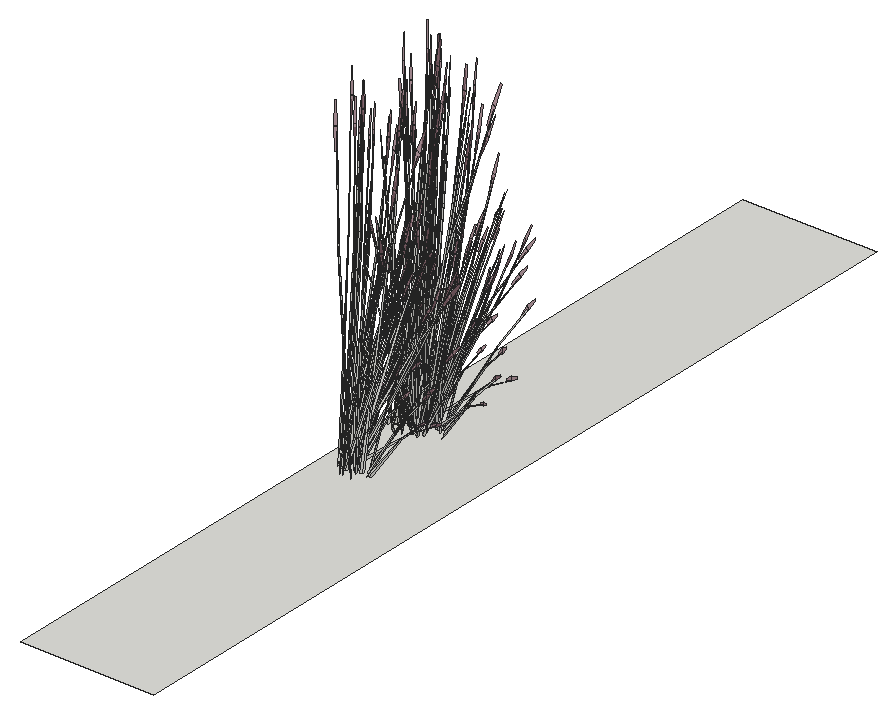
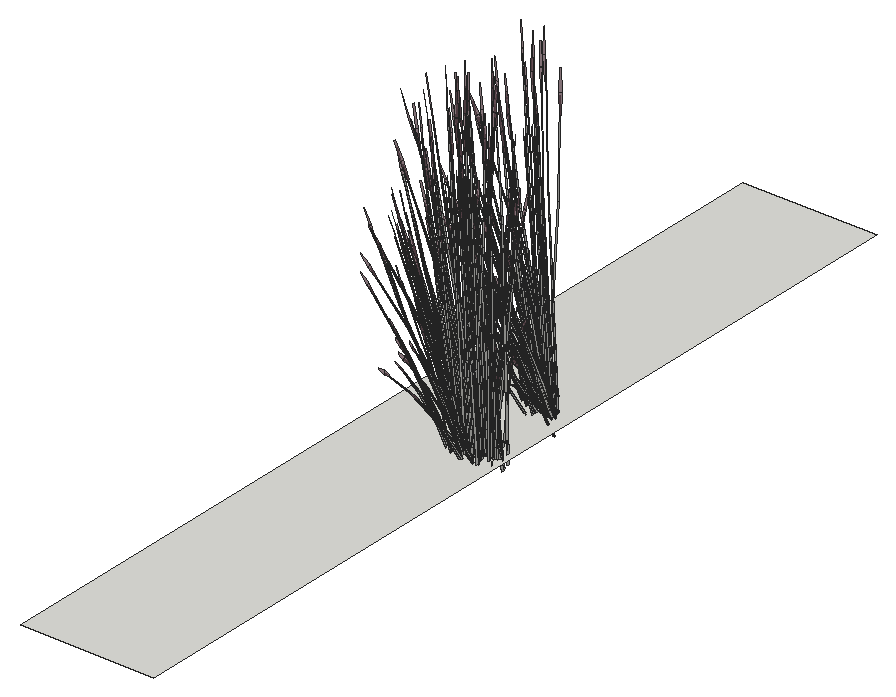
# SketchUp Ruby script. Lengths in inches.
U = 1.inch
M = Sketchup.active_model
def pt(a) = Geom::Point3d.new(a.map { |v| v * U })
def face(e, loops, mat)
  f = e.add_face(loops[0].map { |a| pt(a) })
  loops[1..].each { |l| e.add_face(l.map { |a| pt(a) }).erase! }
  f.material = f.back_material = mat if mat
  f
end
# faces: each face lists its corners as indices into pts; further lists are holes
def faces(e, pts, list, mat = nil) = list.each { |f| face(e, (f[0].is_a?(Array) ? f : [f]).map { |l| l.map { |i| pts[i] } }, mat) }
# xy, xz, yz: faces in a plane at the given z, y or x. An outline is a flat list of corners, or four numbers for a rectangle; further outlines are holes
def ring(l) = l.size == 4 ? [[l[0], l[1]], [l[2], l[1]], [l[2], l[3]], [l[0], l[3]]] : l.each_slice(2).to_a
def flat(e, list, mat, &to3) = list.each { |f| face(e, (f[0].is_a?(Array) ? f : [f]).map { |l| ring(l).map { |u, v| to3.(u, v) } }, mat) }
def xy(e, z, list, mat = nil) = flat(e, list, mat) { |x, y| [x, y, z] }
def xz(e, y, list, mat = nil) = flat(e, list, mat) { |x, z| [x, y, z] }
def yz(e, x, list, mat = nil) = flat(e, list, mat) { |y, z| [x, y, z] }
def lines(e, pts, list) = list.each { |a, b| e.add_line(pt(pts[a]), pt(pts[b])) }
# prism: a flat outline (further loops are holes) pulled along v
def prism(e, loops, v, mat = nil)
  f = face(e, loops, mat); d = Geom::Vector3d.new(v.map { |x| x * U })
  f.pushpull(f.normal.samedirection?(d) ? d.length : -d.length)
end
def box(e, o, s, mat = nil) = prism(e, [[o, [o[0] + s[0], o[1], o[2]], [o[0] + s[0], o[1] + s[1], o[2]], [o[0], o[1] + s[1], o[2]]]], [0, 0, s[2]], mat)
def at(x, y, z, deg = 0) = Geom::Transformation.translation(pt([x, y, z])) * Geom::Transformation.rotation(ORIGIN, Z_AXIS, deg.degrees)
def axes(o, x, y, z) = Geom::Transformation.new([*x, 0, *y, 0, *z, 0, *pt(o).to_a, 1])
def part(name) = M.definitions.add(name)
# library, detail: a bought-in or finely detailed component or shape, given as its bounding box
def library(name, o, s) = part(name).tap { |d| box(d.entities, o, s) }
def detail(e, o, s) = box(e.add_group.entities, o, s)
def put(e, d, t, mat = nil) = e.add_instance(d, t).tap { |i| i.material = mat if mat }
def group(e, t, mat = nil) = e.add_group.tap { |g| g.transformation = t; g.material = mat if mat }.entities
root = M.entities
M.materials.add("LightPink_Translucent").color = [144, 107, 117]
M.materials["LightPink_Translucent"].alpha = 0.75
c1 = part("blade")
p = [[2.15,0.21,22],[0,0.17,0],[0.09,0.45,0],[2.18,0.31,22],[2.29,0.31,22],[0.38,0.45,0],
  [2.48,0.24,33],[2.49,0.24,33],[2.48,0.22,33]]
faces(c1.entities,p,[[0,1,2,3],[4,5,2,3],[6,3,4,7],[8,0,3,6]])
c2 = part("seeds")
p = [[0.3,-0.1,1.38],[-0.01,-0.03,1.59],[-0.01,-0.03,0.03],[0.14,-0.07,-0.07],[0.29,-0.03,3],[0.15,0.01,3.11]]
faces(c2.entities,p,[[0,1,2,3],[1,0,4,5]],"LightPink_Translucent")
c3 = part("blade with seeds")
put(c3.entities,c1,at(0,0,0))
put(c3.entities,c2,axes([2.4,0.25,30.99],[1.5799,-0.05474,1.17369],[-0.12525,1.92788,0.29478],[-0.07173,-0.02425,1.56792]))
xy(root,6,[[342,51,366,213]])
put(root,c3,axes([345.73,119.64,4.48],[0.93921,-0.22138,-0.19198],[0.33003,0.6377,0.00008],[0.10367,-0.02447,1.73897]))
put(root,c3,axes([345.84,118.43,4.51],[0.62448,0.42144,0],[-0.62448,0.42144,0],[0,0,1.69266]))
put(root,c3,axes([347.53,118.25,4.77],[-0.70288,-0.47526,0.17642],[0.70832,-0.46097,0.35086],[-0.07763,0.09706,1.60407]))
put(root,c3,axes([346.23,117.53,4.35],[0.9306,0.10697,-0.62353],[-0.19638,0.65984,-0.16365],[0.27771,0.07995,1.37633]))
put(root,c3,axes([350.34,118.68,5.06],[-0.55274,0.10771,1.1486],[0.26018,-0.44517,0.84392],[0.29323,0.03046,0.25299]))
put(root,c3,axes([345.83,117.9375,5.01],[0.43405,-0.58792,0.44739],[0.90188,0.28295,-0.21531],[0,0.13553,1.43643]))
put(root,c3,axes([350.09,120.57,7],[-0.08089,-0.05712,1.77383],[0.17695,-0.61228,-0.16761],[0.31864,-0.03912,0.31391]))
put(root,c3,axes([345.67,118.28,4.59],[0,0.75458,-0.05637],[-1.11865,0,0],[0,0.02371,1.79368]))
put(root,c3,axes([345.75,117.74,4.5],[0.53742,0.54764,-0.44739],[-0.81403,0.38564,0.21531],[0.17391,0.06776,1.43643]))
put(root,c3,axes([349.38,120.06,6.22],[-0.17122,-0.54847,-0.03492],[0.80929,-0.12609,-0.15832],[0.169,0.03477,0.52218]))
put(root,c3,axes([347.28,120.04,7.33],[0.0479,-0.66354,-0.1216],[0.90696,0.01814,-0.67495],[0.3493,0.04609,1.02557]))
put(root,c3,axes([348.11,118.27,4.77],[0,-0.65246,0.49651],[1.00089,0,0],[0,0.1486,1.57504]))
put(root,c3,axes([346.21,118.07,4.91],[0.83351,-0.19028,0.1448],[0.29189,0.54335,-0.41347],[0,0.11958,1.26744]))
put(root,c3,axes([347.14,119.78,7.34],[-0.50902,-0.40851,0.35414],[0.58122,-0.38671,-0.4572],[0.29531,0.05884,0.87481]))
put(root,c3,axes([349.31,119.4,4.88],[-0.21545,-0.16047,1.43002],[0.28033,-0.53085,-0.30754],[0.43591,0.07191,0.61141]))
put(root,c3,axes([345.45,119.98,4.5],[0.90188,0.29293,0],[-0.43405,0.60866,0],[0,0,1.74954]))
put(root,c3,axes([348.07,119.64,7.01],[0.19191,-0.01103,1.74944],[0.52639,-0.5069,-0.27667],[0.34136,0.06691,0.14031]))
put(root,c3,axes([347.33,119.72,7.27],[0.89428,0.01571,-0.71045],[-0.06006,0.66153,0.08574],[0.37886,0.06981,1.00501]))
put(root,c3,axes([345.13,119.74,4.58],[0.38895,0.74956,-0.06012],[-1.11135,0.26265,0],[0.01358,0.02618,1.72173]))
put(root,c3,axes([348.79,118.38,4.67],[1.11865,0,0],[0,0.72922,-0.51607],[0,0.16609,1.63711]))
put(root,c3,axes([348.34,118.75,4.49],[-1.1181,-0.00522,-0.04976],[0,-0.72922,0.49943],[-0.03514,0.166,1.58352]))
put(root,c3,axes([345.92,118.12,4.96],[1.00749,0.31132,-0.29095],[-0.48511,0.65709,-0.50002],[0.03166,0.16133,1.59708]))
put(root,c3,axes([347.87,119.99,6.82],[0.50902,0.40851,-0.35414],[-0.58122,0.38671,0.4572],[0.29531,0.05884,0.87481]))
put(root,c3,axes([348.11,118.86,4.32],[-0.62448,0.40708,-0.30978],[-0.62448,-0.40708,0.30978],[0,0.13112,1.38974]))
put(root,c3,axes([347.61,120.15,7.02],[-0.04505,0.49615,0.0643],[-0.68022,-0.0136,0.50621],[0.26056,0.05192,0.77189]))
put(root,c3,axes([345.81,118.61,4.5],[-0.43405,0.58792,-0.44739],[-0.90188,-0.28295,0.21531],[0,0.13553,1.43643]))
put(root,c3,axes([347.67,119.99,7.03],[-0.65964,0.42992,0.48003],[-0.5689,-0.45657,0.3958],[0.30948,0.0793,0.9933]))
put(root,c3,axes([345.57,120.49,7.34],[-0.13817,-0.52554,0.35414],[0.78985,-0.13877,-0.4572],[0.21215,0.1506,0.87481]))
put(root,c3,axes([348.54,118.87,4.3125],[0,0.65246,-0.49651],[-1.00089,0,0],[0,0.1486,1.57504]))
put(root,c3,axes([346.04,118.95,6.17],[-0.3323,-0.11241,1.71376],[0.68769,-0.4716,0.13857],[0.42861,0.21275,0.73262]))
put(root,c3,axes([346.1,117.47,6.77],[-0.77304,-0.33901,1.38283],[0.81626,-0.52782,0.59665],[0.24941,0.31809,1.33663]))
put(root,c3,axes([347.27,120.23,5.06],[-0.5037,-0.18761,1.1486],[0.6504,-0.19062,0.84392],[0.17543,0.16147,0.25299]))
put(root,c3,axes([345.5,120.76,7.33],[0.53309,-0.55848,-0.1216],[0.77201,0.32175,-0.67495],[0.26836,0.15779,1.02557]))
put(root,c3,axes([344.8,121.23,7],[0.00265,-0.07899,1.77383],[0.76665,-0.34851,-0.16761],[0.2663,0.12439,0.31391]))
put(root,c3,axes([347.41,120.92,3.79],[0.06518,-0.0942,1.76342],[0.82057,-0.27742,-0.26939],[0.24877,0.14358,0.30037]))
put(root,c3,axes([346.33,118.78,4.39],[0.32803,0.59738,-0.69212],[-0.94492,0.21515,-0.18165],[0.03626,0.20229,1.52773]))
put(root,c3,axes([346.13,120.48,6.97],[0.88277,-0.1551,-0.51099],[0.15442,0.58737,-0.3958],[0.23711,0.16832,0.97773]))
put(root,c3,axes([343.68,120.57,7.34],[0.2697,-0.50175,0.35414],[0.78684,0.14635,-0.4572],[0.07215,0.20201,0.87481]))
put(root,c3,axes([347.35,121.08,4.96],[-0.57368,-0.02046,1.0506],[0.37886,-0.43461,0.58006],[0.22663,0.15441,0.8241]))
put(root,c3,axes([345.7,120.97,7.02],[-0.4066,0.41448,0.0643],[-0.57901,-0.24131,0.50621],[0.18719,0.13288,0.77189]))
put(root,c3,axes([344.74,122.36,7.9375],[0.61821,-0.37431,-0.06488],[0.56645,0.40995,-0.29416],[0.03988,0.11616,0.97024]))
put(root,c3,axes([345.87,120.85,7.03],[-0.88979,0.14973,0.48003],[-0.15442,-0.58737,0.3958],[0.20926,0.17311,0.9933]))
put(root,c3,axes([345.48,120.03,4.88],[0.01579,-0.21629,1.43002],[0.75442,-0.24159,-0.30754],[0.23289,0.25887,0.61141]))
put(root,c3,axes([343.42,120.78,7.33],[0.87543,-0.30377,-0.1216],[0.4302,0.53915,-0.67495],[0.1155,0.2272,1.02557]))
put(root,c3,axes([343.58,120.9,3.79],[0.14478,-0.0355,1.76342],[0.8709,0.19542,-0.26939],[0.02547,0.22025,0.30037]))
put(root,c3,axes([344.17,120.76,6.97],[0.87941,0.16356,-0.51099],[-0.30143,0.56078,-0.3958],[0.08064,0.22578,0.97773]))
put(root,c3,axes([344.67,119.6,6.17],[-0.2045,-0.20949,1.71376],[0.94495,-0.17636,0.13857],[0.21357,0.32887,0.73262]))
put(root,c3,axes([343.77,121.1,6.82],[-0.2697,0.50175,-0.35414],[-0.78684,-0.14635,0.4572],[0.07215,0.20201,0.87481]))
put(root,c3,axes([343.85,120.65,7.27],[0.42698,0.53052,-0.71045],[-0.87893,0.29566,0.08574],[0.09984,0.25633,1.00501]))
put(root,c3,axes([343.21,121.99,7.01],[0.1134,0.10507,1.74944],[0.91515,0.04128,-0.27667],[0.09203,0.23172,0.14031]))
put(root,c3,axes([346.1,132.13,4.88],[-0.25429,0.13207,1.43002],[-0.76157,-0.23115,-0.30754],[0.14117,-0.28747,0.61141]))
put(root,c3,axes([346.72,133.11,7.27],[0.02328,-0.60353,-0.71045],[0.98022,0.04053,0.08574],[0.10344,-0.25568,1.00501]))
put(root,c3,axes([348.09,132.17,7.01],[-0.00864,-0.12985,1.74944],[-0.72937,-0.3753,-0.27667],[0.11277,-0.2275,0.14031]))
put(root,c3,axes([345.62,132.81,6.17],[-0.16657,0.22426,1.71376],[-0.69879,-0.4641,0.13857],[0.31524,-0.28926,0.73262]))
put(root,c3,axes([347.89,131.7,7],[-0.09085,0.04984,1.77383],[-0.89014,-0.16814,-0.16761],[-0.03222,-0.21748,0.31391]))
put(root,c3,axes([345.16,131.08,5.06],[0.11476,0.38047,1.1486],[-0.63664,-0.21072,0.84392],[0.06851,-0.19481,0.25299]))
put(root,c3,axes([346.52,132.91,6.97],[-0.64041,-0.4384,-0.51099],[0.67652,-0.38394,-0.3958],[0.09744,-0.22274,0.97773]))
put(root,c3,axes([345.12,132.26,7.03],[0.88151,0.17057,0.48003],[-0.30143,0.56078,0.3958],[-0.05297,-0.22053,0.9933]))
put(root,c3,axes([347.19,133.14,7.33],[-0.98321,-0.03233,-0.1216],[0.02687,-0.61208,-0.67495],[0.0683,-0.23574,1.02557]))
put(root,c3,axes([347.12,132.75,6.82],[0.60531,-0.34352,-0.35414],[0.573,0.39225,0.4572],[0.08718,-0.19929,0.87481]))
put(root,c3,axes([345.35,132.22,7.02],[0.6592,-0.22175,0.0643],[0.32265,0.40436,0.50621],[-0.06366,-0.17825,0.77189]))
put(root,c3,axes([347.88,132.54,3.79],[-0.1339,-0.0514,1.76342],[-0.34394,-0.57425,-0.26939],[0.23202,-0.15583,0.30037]))
put(root,c3,axes([347.12,132.88,7.03],[0.63704,0.44518,0.48003],[-0.67652,0.38394,0.3958],[0.11751,-0.20886,0.9933]))
put(root,c3,axes([347.36,132.93,7.02],[0.73517,0.0304,0.0643],[-0.02016,0.45906,0.50621],[0.07693,-0.17585,0.77189]))
put(root,c3,axes([346.81,133.24,7.34],[-0.60531,0.34352,0.35414],[-0.573,-0.39225,-0.4572],[0.08718,-0.19929,0.87481]))
put(root,c3,axes([347.875,134.16,7.27],[0.4673,-0.51481,-0.71045],[0.81887,0.36587,0.08574],[0.27902,-0.18652,1.00501]))
put(root,c3,axes([342.82,132.66,4.67],[-0.55932,-0.6538,0],[0.93577,-0.36461,-0.51607],[0.21313,-0.08304,1.63711]))
put(root,c3,axes([347.85,133.92,6.97],[-0.22982,-0.59576,-0.51099],[0.87033,-0.10422,-0.3958],[0.24941,-0.16002,0.97773]))
put(root,c3,axes([348.26,134.35,7.33],[-0.82753,-0.35977,-0.1216],[0.47675,-0.52101,-0.67495],[0.2338,-0.18111,1.02557]))
put(root,c3,axes([343.58,132.5625,4.3125],[0.83726,-0.32623,-0.49651],[0.50045,0.58498,0],[0.19069,-0.0743,1.57504]))
put(root,c3,axes([348.55,133.6875,4.88],[-0.31959,-0.01933,1.43002],[-0.32741,-0.51843,-0.30754],[0.39262,-0.14666,0.61141]))
put(root,c3,axes([350.3,134.19,7],[-0.11685,-0.00496,1.77383],[-0.48522,-0.53096,-0.16761],[0.19486,-0.17458,0.31391]))
put(root,c3,axes([344.57,133.9,4.35],[0.60257,-0.49041,-0.62353],[0.74854,0.44469,-0.16365],[0.24146,-0.12234,1.37633]))
put(root,c3,axes([348.92,132.74,5.06],[-0.29798,0.33213,1.1486],[-0.25612,-0.44624,0.84392],[0.24611,-0.11182,0.25299]))
put(root,c3,axes([348.49,133.98,6.82],[0.77872,-0.09325,-0.35414],[0.20563,0.53305,0.4572],[0.22316,-0.14318,0.87481]))
put(root,c3,axes([343.53,134.76,4.5],[0.43405,-0.58792,-0.44739],[0.90188,0.28295,0.21531],[0,-0.13553,1.43643]))
put(root,c3,axes([343.92,134.47,4.96],[-0.10425,-0.7445,-0.29095],[1.08575,-0.04502,-0.50002],[0.19119,-0.09917,1.59708]))
put(root,c3,axes([347.86,134.3,7.34],[-0.77872,0.09325,0.35414],[-0.20563,-0.53305,-0.4572],[0.22316,-0.14318,0.87481]))
put(root,c3,axes([343.78,132.82,4.32],[0.83462,0.16144,-0.30978],[-0.21015,0.56852,0.30978],[0.16826,-0.06556,1.38974]))
put(root,c3,axes([348.5625,134.21,7.02],[0.61415,0.2744,0.0643],[-0.35756,0.39076,0.50621],[0.1969,-0.12633,0.77189]))
put(root,c3,axes([348.39,134.1,7.03],[0.22187,0.60049,0.48003],[-0.87033,0.10422,0.3958],[0.25651,-0.14123,0.9933]))
put(root,c3,axes([350.74,134.83,7.01],[0.12414,-0.09938,1.74944],[-0.15889,-0.60963,-0.27667],[0.31148,-0.11559,0.14031]))
put(root,c3,axes([344.0625,135.05,4.73],[1.00799,0.31623,0.24065],[-0.48511,0.65709,0.50002],[0,-0.15147,1.60543]))
put(root,c3,axes([343.74,134.61,5.01],[-0.97146,0.04028,0.44739],[-0.08785,-0.66859,-0.21531],[0.17391,-0.06776,1.43643]))
put(root,c3,axes([348.29,135.75,7.33],[-0.45012,-0.59081,-0.1216],[0.79888,-0.29033,-0.67495],[0.33665,-0.07795,1.02557]))
put(root,c3,axes([348.26,135.24,6.97],[0.24236,-0.59349,-0.51099],[0.83094,0.20343,-0.3958],[0.33455,-0.05442,0.97773]))
put(root,c3,axes([346.94,132.83,4.67],[0.55932,-0.6538,0],[0.93577,0.36461,-0.51607],[0.21313,0.08304,1.63711]))
put(root,c3,axes([349.14,135.41,4.28],[-0.57619,0.0783,1.41583],[-0.09171,-0.62326,0.08104],[0.40356,-0.09434,0.80566]))
put(root,c3,axes([350.19,134.86,4.55],[-0.55463,-0.41721,-0.06488],[0.60744,-0.38228,-0.29416],[0.17212,-0.02691,0.97024]))
put(root,c3,axes([345.1,134.91,4.5],[0,-0.75495,0],[1.11865,0,0],[0,0,1.79456]))
put(root,c3,axes([346.46,133.17,4.77],[-0.83726,-0.32623,0.49651],[0.50045,-0.58498,0],[0.19069,0.0743,1.57504]))
put(root,c3,axes([348.1,135.46,7.27],[0.78611,-0.28816,-0.71045],[0.4381,0.59317,0.08574],[0.37982,-0.06738,1.00501]))
put(root,c3,axes([344.57,134.4375,4.65],[-0.74176,0.59212,0.45755],[-0.88124,-0.52269,0.17955],[0.17882,-0.05909,1.58856]))
put(root,c3,axes([343.29,133.46,4.77],[-0.25843,0.64844,0.17642],[-0.9457,-0.1835,0.35086],[0.16336,-0.00316,1.60407]))
put(root,c3,axes([347.98,135.57,7.34],[-0.74348,-0.18202,0.35414],[0.21685,-0.53102,-0.4572],[0.29933,-0.04869,0.87481]))
put(root,c3,axes([342.89,133.99,3.89],[-0.88056,0.26122,1.28929],[-0.28027,-0.74951,0.50096],[0.54072,0.01247,1.46642]))
put(root,c3,axes([345.26,134.18,4.91],[0.17258,-0.58229,0.1448],[0.84319,0.10108,-0.41347],[0.15345,0.05979,1.26744]))
put(root,c3,axes([349.77,135,3.79],[-0.04675,-0.09906,1.76342],[0.32428,-0.57943,-0.26939],[0.32711,-0.00833,0.30037]))
put(root,c3,axes([344.9,134.34,5.01],[-0.53742,-0.54764,0.44739],[0.81403,-0.38564,-0.21531],[0.17391,0.06776,1.43643]))
put(root,c3,axes([345.17,134.375,4.96],[0.90324,-0.43318,-0.29095],[0.60064,0.61207,-0.50002],[0.22285,0.06216,1.59708]))
put(root,c3,axes([348.76,135.52,6.82],[0.74348,0.18202,-0.35414],[-0.21685,0.53102,0.4572],[0.29933,-0.04869,0.87481]))
put(root,c3,axes([347.45,133.22,4.3125],[0.83726,0.32623,-0.49651],[-0.50045,0.58498,0],[0.19069,0.0743,1.57504]))
put(root,c3,axes([345.86,135.08,4.5],[1.00089,0,0],[0,0.67548,0],[0,0,1.78407]))
put(root,c3,axes([346.15,133.5,4.77],[-0.96132,0.17317,0.17642],[-0.23737,-0.64447,0.35086],[0.08574,0.0939,1.60407]))
put(root,c3,axes([346.74,134.86,6.17],[-0.37107,0.01478,1.71376],[0.24616,-0.64047,0.13857],[0.5288,0.03961,0.73262]))
put(root,c3,axes([347.22,133.47,4.32],[0.21015,0.56852,-0.30978],[-0.83462,0.16144,0.30978],[0.16826,0.06556,1.38974]))
put(root,c3,axes([348.66,135.74,7.02],[0.32857,0.44488,0.0643],[-0.59916,0.21775,0.50621],[0.26412,-0.04296,0.77189]))
put(root,c3,axes([345.54,134.74,4.67],[-1.13071,-0.13747,0.49198],[0.23011,-0.77639,0.19306],[0.16524,0.07497,1.70813]))
put(root,c3,axes([348.59,135.58,7.03],[-0.25275,0.59491,0.48003],[-0.83094,-0.20343,0.3958],[0.32677,-0.03575,0.9933]))
put(root,c3,axes([344.64,136.66,4.5],[-0.29189,-0.56252,0],[0.83351,-0.19699,0],[0,0,1.54371]))
put(root,c3,axes([345.73,136.58,4.48],[0.93921,-0.22138,-0.19198],[0.33003,0.6377,0.00008],[0.10367,-0.02447,1.73897]))
put(root,c3,axes([345.84,135.37,4.51],[0.62448,0.42144,0],[-0.62448,0.42144,0],[0,0,1.69266]))
put(root,c3,axes([347.53,135.1875,4.77],[-0.70288,-0.47526,0.17642],[0.70832,-0.46097,0.35086],[-0.07763,0.09706,1.60407]))
put(root,c3,axes([346.23,134.47,4.35],[0.9306,0.10697,-0.62353],[-0.19638,0.65984,-0.16365],[0.27771,0.07995,1.37633]))
put(root,c3,axes([350.34,135.625,5.06],[-0.55274,0.10771,1.1486],[0.26018,-0.44517,0.84392],[0.29323,0.03046,0.25299]))
put(root,c3,axes([345.83,134.88,5.01],[0.43405,-0.58792,0.44739],[0.90188,0.28295,-0.21531],[0,0.13553,1.43643]))
put(root,c3,axes([350.09,137.51,7],[-0.08089,-0.05712,1.77383],[0.17695,-0.61228,-0.16761],[0.31864,-0.03912,0.31391]))
put(root,c3,axes([345.67,135.22,4.59],[0,0.75458,-0.05637],[-1.11865,0,0],[0,0.02371,1.79368]))
put(root,c3,axes([345.75,134.68,4.5],[0.53742,0.54764,-0.44739],[-0.81403,0.38564,0.21531],[0.17391,0.06776,1.43643]))
put(root,c3,axes([349.38,137,6.22],[-0.17122,-0.54847,-0.03492],[0.80929,-0.12609,-0.15832],[0.169,0.03477,0.52218]))
put(root,c3,axes([347.28,136.98,7.33],[0.0479,-0.66354,-0.1216],[0.90696,0.01814,-0.67495],[0.3493,0.04609,1.02557]))
put(root,c3,axes([348.11,135.21,4.77],[0,-0.65246,0.49651],[1.00089,0,0],[0,0.1486,1.57504]))
put(root,c3,axes([346.21,135.01,4.91],[0.83351,-0.19028,0.1448],[0.29189,0.54335,-0.41347],[0,0.11958,1.26744]))
put(root,c3,axes([347.14,136.72,7.34],[-0.50902,-0.40851,0.35414],[0.58122,-0.38671,-0.4572],[0.29531,0.05884,0.87481]))
put(root,c3,axes([349.31,136.34,4.88],[-0.21545,-0.16047,1.43002],[0.28033,-0.53085,-0.30754],[0.43591,0.07191,0.61141]))
put(root,c3,axes([345.45,136.92,4.5],[0.90188,0.29293,0],[-0.43405,0.60866,0],[0,0,1.74954]))
put(root,c3,axes([348.07,136.58,7.01],[0.19191,-0.01103,1.74944],[0.52639,-0.5069,-0.27667],[0.34136,0.06691,0.14031]))
put(root,c3,axes([347.33,136.66,7.27],[0.89428,0.01571,-0.71045],[-0.06006,0.66153,0.08574],[0.37886,0.06981,1.00501]))
put(root,c3,axes([345.13,136.68,4.58],[0.38895,0.74956,-0.06012],[-1.11135,0.26265,0],[0.01358,0.02618,1.72173]))
put(root,c3,axes([348.79,135.32,4.67],[1.11865,0,0],[0,0.72922,-0.51607],[0,0.16609,1.63711]))
put(root,c3,axes([348.34,135.69,4.49],[-1.1181,-0.00522,-0.04976],[0,-0.72922,0.49943],[-0.03514,0.166,1.58352]))
put(root,c3,axes([345.92,135.06,4.96],[1.00749,0.31132,-0.29095],[-0.48511,0.65709,-0.50002],[0.03166,0.16133,1.59708]))
put(root,c3,axes([347.87,136.93,6.82],[0.50902,0.40851,-0.35414],[-0.58122,0.38671,0.4572],[0.29531,0.05884,0.87481]))
put(root,c3,axes([348.11,135.8,4.32],[-0.62448,0.40708,-0.30978],[-0.62448,-0.40708,0.30978],[0,0.13112,1.38974]))
put(root,c3,axes([347.61,137.09,7.02],[-0.04505,0.49615,0.0643],[-0.68022,-0.0136,0.50621],[0.26056,0.05192,0.77189]))
put(root,c3,axes([345.81,135.55,4.5],[-0.43405,0.58792,-0.44739],[-0.90188,-0.28295,0.21531],[0,0.13553,1.43643]))
put(root,c3,axes([347.67,136.93,7.03],[-0.65964,0.42992,0.48003],[-0.5689,-0.45657,0.3958],[0.30948,0.0793,0.9933]))
put(root,c3,axes([345.57,137.43,7.34],[-0.13817,-0.52554,0.35414],[0.78985,-0.13877,-0.4572],[0.21215,0.1506,0.87481]))
put(root,c3,axes([348.54,135.8125,4.3125],[0,0.65246,-0.49651],[-1.00089,0,0],[0,0.1486,1.57504]))
put(root,c3,axes([346.04,135.89,6.17],[-0.3323,-0.11241,1.71376],[0.68769,-0.4716,0.13857],[0.42861,0.21275,0.73262]))
put(root,c3,axes([346.1,134.41,6.77],[-0.77304,-0.33901,1.38283],[0.81626,-0.52782,0.59665],[0.24941,0.31809,1.33663]))
put(root,c3,axes([347.27,137.17,5.06],[-0.5037,-0.18761,1.1486],[0.6504,-0.19062,0.84392],[0.17543,0.16147,0.25299]))
put(root,c3,axes([345.5,137.7,7.33],[0.53309,-0.55848,-0.1216],[0.77201,0.32175,-0.67495],[0.26836,0.15779,1.02557]))
put(root,c3,axes([344.8,138.17,7],[0.00265,-0.07899,1.77383],[0.76665,-0.34851,-0.16761],[0.2663,0.12439,0.31391]))
